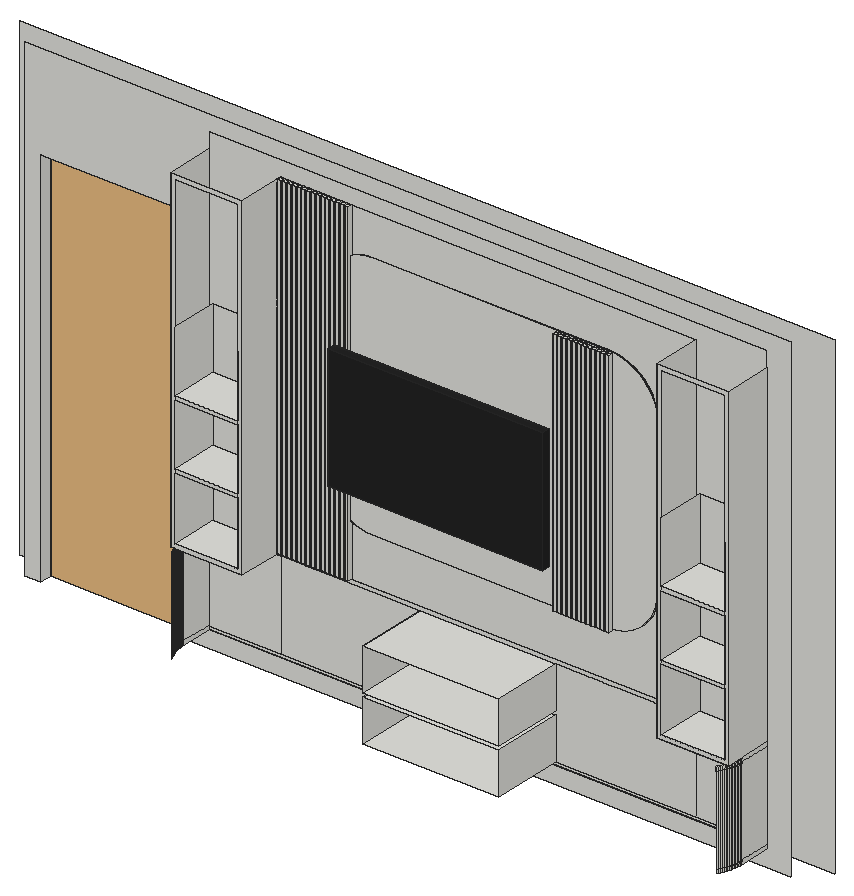
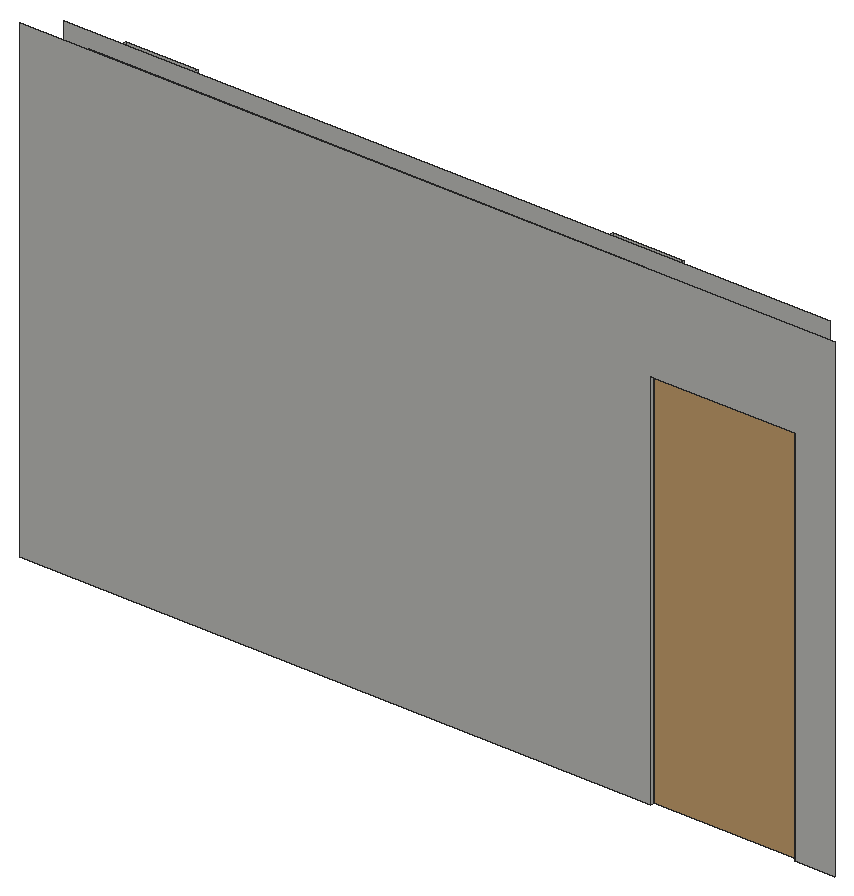
# SketchUp Ruby script. Lengths in inches.
U = 1.inch
M = Sketchup.active_model
def pt(a) = Geom::Point3d.new(a.map { |v| v * U })
def face(e, loops, mat)
  f = e.add_face(loops[0].map { |a| pt(a) })
  loops[1..].each { |l| e.add_face(l.map { |a| pt(a) }).erase! }
  f.material = f.back_material = mat if mat
  f
end
# faces: each face lists its corners as indices into pts; further lists are holes
def faces(e, pts, list, mat = nil) = list.each { |f| face(e, (f[0].is_a?(Array) ? f : [f]).map { |l| l.map { |i| pts[i] } }, mat) }
# xy, xz, yz: faces in a plane at the given z, y or x. An outline is a flat list of corners, or four numbers for a rectangle; further outlines are holes
def ring(l) = l.size == 4 ? [[l[0], l[1]], [l[2], l[1]], [l[2], l[3]], [l[0], l[3]]] : l.each_slice(2).to_a
def flat(e, list, mat, &to3) = list.each { |f| face(e, (f[0].is_a?(Array) ? f : [f]).map { |l| ring(l).map { |u, v| to3.(u, v) } }, mat) }
def xy(e, z, list, mat = nil) = flat(e, list, mat) { |x, y| [x, y, z] }
def xz(e, y, list, mat = nil) = flat(e, list, mat) { |x, z| [x, y, z] }
def yz(e, x, list, mat = nil) = flat(e, list, mat) { |y, z| [x, y, z] }
def lines(e, pts, list) = list.each { |a, b| e.add_line(pt(pts[a]), pt(pts[b])) }
# prism: a flat outline (further loops are holes) pulled along v
def prism(e, loops, v, mat = nil)
  f = face(e, loops, mat); d = Geom::Vector3d.new(v.map { |x| x * U })
  f.pushpull(f.normal.samedirection?(d) ? d.length : -d.length)
end
def box(e, o, s, mat = nil) = prism(e, [[o, [o[0] + s[0], o[1], o[2]], [o[0] + s[0], o[1] + s[1], o[2]], [o[0], o[1] + s[1], o[2]]]], [0, 0, s[2]], mat)
def at(x, y, z, deg = 0) = Geom::Transformation.translation(pt([x, y, z])) * Geom::Transformation.rotation(ORIGIN, Z_AXIS, deg.degrees)
def axes(o, x, y, z) = Geom::Transformation.new([*x, 0, *y, 0, *z, 0, *pt(o).to_a, 1])
def part(name) = M.definitions.add(name)
# library, detail: a bought-in or finely detailed component or shape, given as its bounding box
def library(name, o, s) = part(name).tap { |d| box(d.entities, o, s) }
def detail(e, o, s) = box(e.add_group.entities, o, s)
def put(e, d, t, mat = nil) = e.add_instance(d, t).tap { |i| i.material = mat if mat }
def group(e, t, mat = nil) = e.add_group.tap { |g| g.transformation = t; g.material = mat if mat }.entities
root = M.entities
M.materials.add("[0136_Charcoal]").color = [35, 35, 35]
c1 = part("Vertical batten \#2")
box(c1.entities,[0,-1,12.125],[1,1,62.125])
c2 = part("Vertical batten \#1")
box(c2.entities,[0,-1,0],[1,1,84])
c3 = library("main+door",[0,-0.79,0],[47.24,7.88,82.68])
xy(root,-59.65,[[567.52,914.04,601.52,932.04]])
xy(root,-49.15,[[567.52,914.04,601.52,932.04]])
xy(root,-48.15,[[567.52,914.04,601.52,932.04]])
xy(root,-37.65,[[567.52,914.04,601.52,932.04]])
xy(root,-36.65,[[514.52,920.04,514.52,924.04,514.53,923.64,514.55,923.25,514.59,922.86,514.64,922.47,514.71,922.09,514.8,921.7,514.9,921.32,515.01,920.95,515.14,920.57,515.28,920.21,515.36,920.04],[515.36,920.04,532.52,920.04,532.52,932.04,514.52,932.04,514.52,924.04,514.53,923.64,514.55,923.25,514.59,922.86,514.64,922.47,514.71,922.09,514.8,921.7,514.9,921.32,515.01,920.95,515.14,920.57,515.28,920.21],[636.52,920.04,653.68,920.04,653.76,920.21,653.9,920.57,654.03,920.95,654.15,921.32,654.24,921.7,654.33,922.09,654.4,922.47,654.45,922.86,654.49,923.25,654.51,923.64,654.52,924.04,654.52,932.04,636.52,932.04],[653.68,920.04,653.76,920.21,653.9,920.57,654.03,920.95,654.15,921.32,654.24,921.7,654.33,922.09,654.4,922.47,654.45,922.86,654.49,923.25,654.51,923.64,654.52,924.04,654.52,920.04]])
xy(root,-35.65,[[515.52,920.04,531.52,932.04],[637.52,920.04,653.52,932.04]])
xy(root,-24.52,[[555.98,931.54,615.33,932.04]])
xy(root,-19.75,[[515.52,920.04,531.52,932.04],[637.52,920.04,653.52,932.04]])
xy(root,-18.75,[[515.52,920.04,531.52,932.04],[637.52,920.04,653.52,932.04]])
xy(root,-3.35,[[515.52,920.04,531.52,932.04],[637.52,920.04,653.52,932.04]])
xy(root,-2.35,[[515.52,920.04,531.52,932.04],[637.52,920.04,653.52,932.04]])
xz(root,920.04,[[[514.52,-36.65,532.52,47.35],[515.52,-35.65,531.52,46.35]],[[636.52,-36.65,654.52,47.35],[637.52,-35.65,653.52,46.35]],[515.52,-19.75,531.52,-18.75],[637.52,-19.75,653.52,-18.75],[515.52,-3.35,531.52,-2.35],
  [637.52,-3.35,653.52,-2.35]])
xz(root,931.54,[[555.98,-24.52,615.33,-24.52,616.9,-24.42,618.4375,-24.11,619.93,-23.61,621.33,-22.91,622.64,-22.04,623.82,-21.01,624.85,-19.83,625.73,-18.52,626.42,-17.11,626.92,-15.625,627.23,-14.09,627.33,-12.52,627.33,25.6,627.23,27.17,626.92,28.71,626.42,30.2,625.73,31.6,624.85,32.91,623.82,34.09,622.64,35.125,621.33,36,619.93,36.69,618.4375,37.2,616.9,37.5,615.33,37.6,555.98,37.6,554.41,37.5,552.875,37.2,551.39,36.69,549.98,36,548.67,35.125,547.49,34.09,546.46,32.91,545.59,31.6,544.89,30.2,544.39,28.71,544.08,27.17,543.98,25.6,543.98,-12.52,544.08,-14.09,544.39,-15.625,544.89,-17.11,545.59,-18.52,546.46,-19.83,547.49,-21.01,548.67,-22.04,549.98,-22.91,551.39,-23.61,552.875,-24.11,554.41,-24.42]])
xz(root,932.04,[[[468.52,-64.65,472.52,-64.65,472.52,31.35,508.52,31.35,508.52,-64.65,660.52,-64.65,660.52,55.35,468.52,55.35],[514.52,-60.65,654.52,51.35]],[514.52,-59.65,532.52,-37.65],[532.52,-59.65,532.52,-37.65,567.52,-37.65,567.52,-48.15,601.52,-48.15,601.52,-37.65,636.52,-37.65,636.52,-59.65,601.52,-59.65,601.52,-49.15,567.52,-49.15,567.52,-59.65],[636.52,-59.65,654.52,-37.65],[514.52,-37.65,532.52,-36.65],
  [532.52,-37.65,636.52,-36.65],[636.52,-37.65,654.52,-36.65],[[533.52,-36.65,636.52,47.35],[555.98,-24.52,554.41,-24.42,552.875,-24.11,551.39,-23.61,549.98,-22.91,548.67,-22.04,547.49,-21.01,546.46,-19.83,545.59,-18.52,544.89,-17.11,544.39,-15.625,544.08,-14.09,543.98,-12.52,543.98,25.6,544.08,27.17,544.39,28.71,544.89,30.2,545.59,31.6,546.46,32.91,547.49,34.09,548.67,35.125,549.98,36,551.39,36.69,552.875,37.2,554.41,37.5,555.98,37.6,615.33,37.6,616.9,37.5,618.4375,37.2,619.93,36.69,621.33,36,622.64,35.125,623.82,34.09,624.85,32.91,625.73,31.6,626.42,30.2,626.92,28.71,627.23,27.17,627.33,25.6,627.33,-12.52,627.23,-14.09,626.92,-15.625,626.42,-17.11,625.73,-18.52,624.85,-19.83,623.82,-21.01,622.64,-22.04,621.33,-22.91,619.93,-23.61,618.4375,-24.11,616.9,-24.42,615.33,-24.52]],[515.52,-35.65,531.52,-19.75],[637.52,-35.65,653.52,-19.75],
  [515.52,-18.75,531.52,-3.35],[637.52,-18.75,653.52,-3.35],[515.52,-2.35,531.52,13.05],[637.52,-2.35,653.52,13.05]])
xz(root,938.04,[[462.52,-64.65,472.52,-64.65,472.52,31.35,508.52,31.35,508.52,-64.65,666.52,-64.65,666.52,55.35,462.52,55.35]])
yz(root,472.52,[[932.04,-64.65,938.04,31.35]])
yz(root,508.52,[[932.04,-64.65,938.04,31.35]])
yz(root,514.52,[[924.04,-60.65,932.04,-59.65],[924.04,-59.65,932.04,-37.65],[924.04,-37.65,932.04,-36.65],[920.04,-36.65,932.04,47.35]])
yz(root,515.52,[[920.04,-35.65,932.04,-19.75],[920.04,-18.75,932.04,-3.35],[920.04,-2.35,932.04,13.05]])
yz(root,531.52,[[920.04,-35.65,932.04,-19.75],[920.04,-18.75,932.04,-3.35],[920.04,-2.35,932.04,13.05]])
yz(root,532.52,[[920.04,-36.65,932.04,47.35]])
yz(root,543.98,[[931.54,-12.52,932.04,25.6]])
yz(root,567.52,[[914.04,-59.65,932.04,-49.15],[914.04,-48.15,932.04,-37.65]])
yz(root,601.52,[[914.04,-59.65,932.04,-49.15],[914.04,-48.15,932.04,-37.65]])
yz(root,627.33,[[931.54,-12.52,932.04,25.6]])
yz(root,636.52,[[920.04,-36.65,932.04,47.35]])
yz(root,637.52,[[920.04,-35.65,932.04,-19.75],[920.04,-18.75,932.04,-3.35],[920.04,-2.35,932.04,13.05]])
yz(root,653.52,[[920.04,-35.65,932.04,-19.75],[920.04,-18.75,932.04,-3.35],[920.04,-2.35,932.04,13.05]])
yz(root,654.52,[[924.04,-60.65,932.04,-59.65],[924.04,-59.65,932.04,-37.65],[924.04,-37.65,932.04,-36.65],[920.04,-36.65,932.04,47.35]])
p = [[516.21,918.48,-60.65],[516.21,918.48,-59.65],[515.99,918.8125,-59.65],[515.99,918.8125,-60.65],[653.05,918.8125,-60.65],[653.05,918.8125,-59.65],
  [652.94,918.65,-59.65],[652.84,918.48,-59.65],[652.84,918.48,-60.65],[515.8,919.15,-59.65],[515.8,919.15,-60.65],[653.25,919.15,-60.65],
  [653.25,919.15,-59.65],[515.61,919.5,-59.65],[515.61,919.5,-60.65],[653.43,919.5,-60.65],[653.43,919.5,-59.65],[515.44,919.85,-59.65],
  [515.44,919.85,-60.65],[653.6,919.85,-60.65],[653.6,919.85,-59.65],[515.28,920.21,-59.65],[515.28,920.21,-60.65],[653.76,920.21,-60.65],
  [653.76,920.21,-59.65],[515.14,920.57,-59.65],[515.14,920.57,-60.65],[653.9,920.57,-60.65],[653.9,920.57,-59.65],[515.01,920.95,-59.65],
  [515.01,920.95,-60.65],[654.03,920.95,-60.65],[654.03,920.95,-59.65],[514.9,921.32,-59.65],[514.9,921.32,-60.65],[654.15,921.32,-60.65],
  [654.15,921.32,-59.65],[514.8,921.7,-59.65],[514.8,921.7,-60.65],[654.24,921.7,-60.65],[654.24,921.7,-59.65],[514.71,922.09,-59.65],
  [514.71,922.09,-60.65],[654.33,922.09,-60.65],[654.33,922.09,-59.65],[514.64,922.47,-59.65],[514.64,922.47,-60.65],[654.4,922.47,-60.65],
  [654.4,922.47,-59.65],[514.59,922.86,-59.65],[514.59,922.86,-60.65],[654.45,922.86,-60.65],[654.45,922.86,-59.65],[514.55,923.25,-59.65],
  [514.55,923.25,-60.65],[654.49,923.25,-60.65],[654.49,923.25,-59.65],[514.53,923.64,-59.65],[514.53,923.64,-60.65],[654.51,923.64,-60.65],
  [654.51,923.64,-59.65],[514.52,924.04,-59.65],[514.52,924.04,-60.65],[654.52,924.04,-60.65],[654.52,924.04,-59.65],[516.21,918.48,-37.65],
  [515.99,918.8125,-37.65],[652.94,918.65,-37.65],[652.84,918.48,-37.65],[653.05,918.8125,-37.65],[515.8,919.15,-37.65],[653.25,919.15,-37.65],
  [515.61,919.5,-37.65],[653.43,919.5,-37.65],[515.44,919.85,-37.65],[653.6,919.85,-37.65],[515.28,920.21,-37.65],[653.76,920.21,-37.65],
  [515.14,920.57,-37.65],[653.9,920.57,-37.65],[515.01,920.95,-37.65],[654.03,920.95,-37.65],[514.9,921.32,-37.65],[654.15,921.32,-37.65],
  [514.8,921.7,-37.65],[654.24,921.7,-37.65],[514.71,922.09,-37.65],[654.33,922.09,-37.65],[514.64,922.47,-37.65],[654.4,922.47,-37.65],
  [514.59,922.86,-37.65],[654.45,922.86,-37.65],[514.55,923.25,-37.65],[654.49,923.25,-37.65],[514.53,923.64,-37.65],[654.51,923.64,-37.65],
  [514.52,924.04,-37.65],[654.52,924.04,-37.65],[516.43,918.16,-36.65],[516.21,918.48,-36.65],[516.43,918.16,-37.65],[652.84,918.48,-36.65],
  [652.61,918.16,-36.65],[652.61,918.16,-37.65],[515.99,918.8125,-36.65],[653.05,918.8125,-36.65],[515.8,919.15,-36.65],[653.25,919.15,-36.65],
  [515.61,919.5,-36.65],[653.43,919.5,-36.65],[515.44,919.85,-36.65],[653.6,919.85,-36.65],[515.36,920.04,-36.65],[515.28,920.21,-36.65],
  [653.68,920.04,-36.65],[653.76,920.21,-36.65],[515.14,920.57,-36.65],[653.9,920.57,-36.65],[515.01,920.95,-36.65],[654.03,920.95,-36.65],
  [514.9,921.32,-36.65],[654.15,921.32,-36.65],[514.8,921.7,-36.65],[654.24,921.7,-36.65],[514.71,922.09,-36.65],[654.33,922.09,-36.65],
  [514.64,922.47,-36.65],[654.4,922.47,-36.65],[514.59,922.86,-36.65],[654.45,922.86,-36.65],[514.55,923.25,-36.65],[654.49,923.25,-36.65],
  [514.53,923.64,-36.65],[654.51,923.64,-36.65],[514.52,924.04,-36.65],[654.52,924.04,-36.65],[554.41,932.04,-24.42],[555.98,932.04,-24.52],
  [555.98,931.54,-24.52],[554.41,931.54,-24.42],[615.33,932.04,-24.52],[616.9,932.04,-24.42],[616.9,931.54,-24.42],[615.33,931.54,-24.52],
  [552.875,932.04,-24.11],[552.875,931.54,-24.11],[618.4375,932.04,-24.11],[618.4375,931.54,-24.11],[551.39,932.04,-23.61],[551.39,931.54,-23.61],
  [619.93,932.04,-23.61],[619.93,931.54,-23.61],[549.98,932.04,-22.91],[549.98,931.54,-22.91],[621.33,932.04,-22.91],[621.33,931.54,-22.91],
  [548.67,932.04,-22.04],[548.67,931.54,-22.04],[622.64,932.04,-22.04],[622.64,931.54,-22.04],[547.49,932.04,-21.01],[547.49,931.54,-21.01],
  [623.82,932.04,-21.01],[623.82,931.54,-21.01],[546.46,932.04,-19.83],[546.46,931.54,-19.83],[624.85,932.04,-19.83],[624.85,931.54,-19.83],
  [545.59,932.04,-18.52],[545.59,931.54,-18.52],[625.73,932.04,-18.52],[625.73,931.54,-18.52],[544.89,932.04,-17.11],[544.89,931.54,-17.11],
  [626.42,932.04,-17.11],[626.42,931.54,-17.11],[544.39,932.04,-15.625],[544.39,931.54,-15.625],[626.92,932.04,-15.625],[626.92,931.54,-15.625],
  [544.08,932.04,-14.09],[544.08,931.54,-14.09],[627.23,932.04,-14.09],[627.23,931.54,-14.09],[543.98,932.04,-12.52],[543.98,931.54,-12.52],
  [627.33,932.04,-12.52],[627.33,931.54,-12.52],[653.52,919.67,-37.65],[653.52,919.67,-59.65]]
faces(root,p,[[0,1,2,3],[4,5,6,7,8],[3,2,9,10],[11,12,5,4],[10,9,13,14],[15,16,12,11],[14,13,17,18],[19,20,16,15],
  [18,17,21,22],[23,24,20,19],[22,21,25,26],[27,28,24,23],[26,25,29,30],[31,32,28,27],[30,29,33,34],[35,36,32,31],
  [34,33,37,38],[39,40,36,35],[38,37,41,42],[43,44,40,39],[42,41,45,46],[47,48,44,43],[46,45,49,50],[51,52,48,47],
  [50,49,53,54],[55,56,52,51],[54,53,57,58],[59,60,56,55],[58,57,61,62],[63,64,60,59],[1,65,66,2],[7,6,67,68],
  [69,67,6,5],[2,66,70,9],[12,71,69,5],[9,70,72,13],[16,73,71,12],[13,72,74,17],[20,75,73,16],[17,74,76,21],
  [24,77,75,20],[21,76,78,25],[28,79,77,24],[25,78,80,29],[32,81,79,28],[29,80,82,33],[36,83,81,32],[33,82,84,37],
  [40,85,83,36],[37,84,86,41],[44,87,85,40],[41,86,88,45],[48,89,87,44],[45,88,90,49],[52,91,89,48],[49,90,92,53],
  [56,93,91,52],[53,92,94,57],[60,95,93,56],[57,94,96,61],[64,97,95,60],[98,99,65,100],[101,102,103,68],[99,104,66,65],
  [105,101,68,67,69],[104,106,70,66],[107,105,69,71],[106,108,72,70],[109,107,71,73],[108,110,74,72],[111,109,73,75],[112,113,76,74,110],
  [114,111,75,77,115],[113,116,78,76],[117,115,77,79],[116,118,80,78],[119,117,79,81],[118,120,82,80],[121,119,81,83],[120,122,84,82],
  [123,121,83,85],[122,124,86,84],[125,123,85,87],[124,126,88,86],[127,125,87,89],[126,128,90,88],[129,127,89,91],[128,130,92,90],
  [131,129,91,93],[130,132,94,92],[133,131,93,95],[132,134,96,94],[135,133,95,97],[136,137,138,139],[140,141,142,143],[144,136,139,145],
  [141,146,147,142],[148,144,145,149],[146,150,151,147],[152,148,149,153],[150,154,155,151],[156,152,153,157],[154,158,159,155],[160,156,157,161],
  [158,162,163,159],[164,160,161,165],[162,166,167,163],[168,164,165,169],[166,170,171,167],[172,168,169,173],[170,174,175,171],[176,172,173,177],
  [174,178,179,175],[180,176,177,181],[178,182,183,179],[184,180,181,185],[182,186,187,183]])
lines(root,p,[[188,189]])
g1 = group(root,at(606.78,921.36,-10.17),"[0136_Charcoal]")
xy(g1,0,[[-53.875,0,0,2]])
xy(g1,15.39,[[-32.58,2,-22.95,5]])
xy(g1,19.08,[[-32.58,2,-22.95,5]])
xy(g1,30.8125,[[-53.875,0,0,2]])
xz(g1,0,[[-53.875,0,0,30.8125]])
xz(g1,2,[[[-53.875,0,0,30.8125],[-32.58,15.39,-22.95,19.08]]])
xz(g1,5,[[-32.58,15.39,-22.95,19.08]])
yz(g1,-53.875,[[0,0,2,30.8125]])
yz(g1,-32.58,[[2,15.39,5,19.08]])
yz(g1,-22.95,[[2,15.39,5,19.08]])
yz(g1,0,[[0,0,2,30.8125]])
put(root,c1,at(602.27,931.04,-36.65))
put(root,c1,at(603.47,931.04,-36.65))
put(root,c1,at(604.67,931.04,-36.65))
put(root,c1,at(605.87,931.04,-36.65))
put(root,c1,at(607.07,931.04,-36.65))
put(root,c1,at(608.27,931.04,-36.65))
put(root,c1,at(609.47,931.04,-36.65))
put(root,c1,at(610.67,931.04,-36.65))
put(root,c1,at(611.87,931.04,-36.65))
put(root,c1,at(613.07,931.04,-36.65))
put(root,c1,at(614.27,931.04,-36.65))
put(root,c1,at(615.47,931.04,-36.65))
put(root,c2,at(532.52,932.04,-36.65))
put(root,c2,at(533.72,932.04,-36.65))
put(root,c2,at(534.92,932.04,-36.65))
put(root,c2,at(536.12,932.04,-36.65))
put(root,c2,at(537.32,932.04,-36.65))
put(root,c2,at(538.52,932.04,-36.65))
put(root,c2,at(539.72,932.04,-36.65))
put(root,c2,at(540.92,932.04,-36.65))
put(root,c2,at(542.12,932.04,-36.65))
put(root,c2,at(543.32,932.04,-36.65))
put(root,c2,at(544.52,932.04,-36.65))
put(root,c2,at(545.72,932.04,-36.65))
put(root,c2,at(546.92,932.04,-36.65))
put(root,c2,at(548.12,932.04,-36.65))
put(root,c2,at(549.32,932.04,-36.65))
put(root,c3,axes([472.55,935.35,-64.65],[0.76132,0,0],[0,0.2584,0],[0,0,1.16114]))
